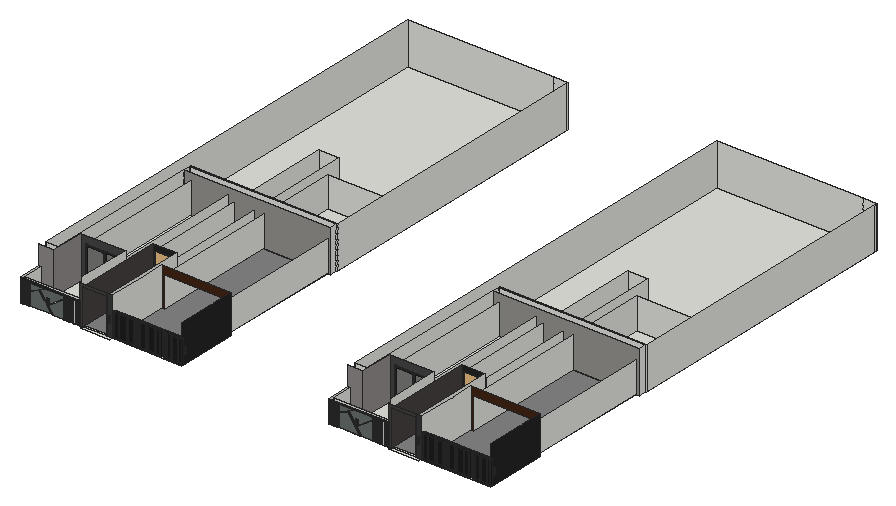
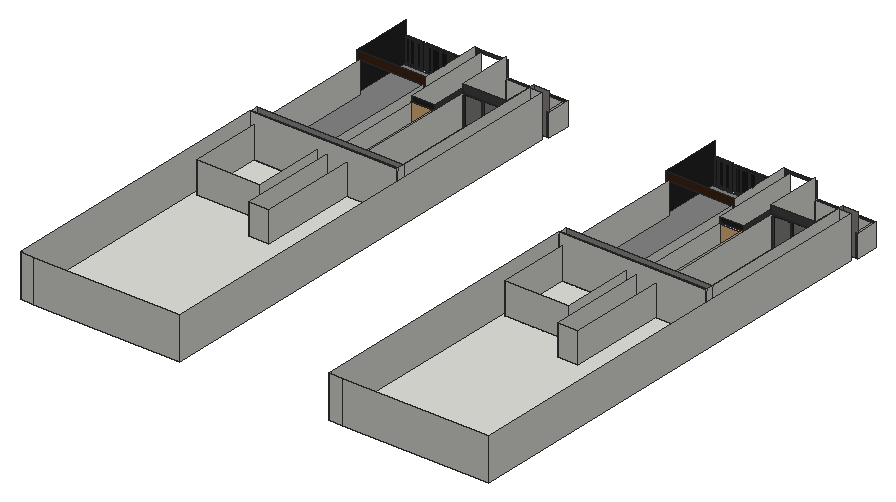
# SketchUp Ruby script. Lengths in inches.
U = 1.inch
M = Sketchup.active_model
def pt(a) = Geom::Point3d.new(a.map { |v| v * U })
def face(e, loops, mat)
  f = e.add_face(loops[0].map { |a| pt(a) })
  loops[1..].each { |l| e.add_face(l.map { |a| pt(a) }).erase! }
  f.material = f.back_material = mat if mat
  f
end
# faces: each face lists its corners as indices into pts; further lists are holes
def faces(e, pts, list, mat = nil) = list.each { |f| face(e, (f[0].is_a?(Array) ? f : [f]).map { |l| l.map { |i| pts[i] } }, mat) }
# xy, xz, yz: faces in a plane at the given z, y or x. An outline is a flat list of corners, or four numbers for a rectangle; further outlines are holes
def ring(l) = l.size == 4 ? [[l[0], l[1]], [l[2], l[1]], [l[2], l[3]], [l[0], l[3]]] : l.each_slice(2).to_a
def flat(e, list, mat, &to3) = list.each { |f| face(e, (f[0].is_a?(Array) ? f : [f]).map { |l| ring(l).map { |u, v| to3.(u, v) } }, mat) }
def xy(e, z, list, mat = nil) = flat(e, list, mat) { |x, y| [x, y, z] }
def xz(e, y, list, mat = nil) = flat(e, list, mat) { |x, z| [x, y, z] }
def yz(e, x, list, mat = nil) = flat(e, list, mat) { |y, z| [x, y, z] }
def lines(e, pts, list) = list.each { |a, b| e.add_line(pt(pts[a]), pt(pts[b])) }
# prism: a flat outline (further loops are holes) pulled along v
def prism(e, loops, v, mat = nil)
  f = face(e, loops, mat); d = Geom::Vector3d.new(v.map { |x| x * U })
  f.pushpull(f.normal.samedirection?(d) ? d.length : -d.length)
end
def box(e, o, s, mat = nil) = prism(e, [[o, [o[0] + s[0], o[1], o[2]], [o[0] + s[0], o[1] + s[1], o[2]], [o[0], o[1] + s[1], o[2]]]], [0, 0, s[2]], mat)
def at(x, y, z, deg = 0) = Geom::Transformation.translation(pt([x, y, z])) * Geom::Transformation.rotation(ORIGIN, Z_AXIS, deg.degrees)
def axes(o, x, y, z) = Geom::Transformation.new([*x, 0, *y, 0, *z, 0, *pt(o).to_a, 1])
def part(name) = M.definitions.add(name)
# library, detail: a bought-in or finely detailed component or shape, given as its bounding box
def library(name, o, s) = part(name).tap { |d| box(d.entities, o, s) }
def detail(e, o, s) = box(e.add_group.entities, o, s)
def put(e, d, t, mat = nil) = e.add_instance(d, t).tap { |i| i.material = mat if mat }
def group(e, t, mat = nil) = e.add_group.tap { |g| g.transformation = t; g.material = mat if mat }.entities
root = M.entities
M.materials.add("Glass_Tinted_Gray").color = [0, 0, 0]
M.materials["Glass_Tinted_Gray"].alpha = 0.125
M.materials.add("[0135_DarkGray]").color = [81, 81, 81]
M.materials.add("[Color M07]").color = [58, 58, 58]
M.materials.add("[Color M08]").color = [30, 30, 30]
M.materials.add("[Granite Dark Gray]").color = [38, 37, 37]
M.materials.add("[Granite Dark Gray]1").color = [69, 68, 68]
M.materials.add("[Granite Light Gray]").color = [149, 148, 144]
M.materials.add("[Granite Tile]1").color = [68, 65, 63]
M.materials.add("[Mirror 02]").color = [229, 229, 229]
M.materials.add("[Slate]").color = [102, 110, 108]
M.materials.add("[Stone Marble]").color = [143, 138, 136]
M.materials.add("[Terrazzo Light Blue]").color = [196, 214, 227]
M.materials.add("[Tile Grey]").color = [132, 132, 132]
M.materials.add("[Wood Veneer 01]").color = [66, 38, 20]
c1 = part("Group\#7")
xy(c1.entities,0,[[6,0,4.45,0.2,3,0.8,1.76,1.76,0.8,3,0.2,4.45,0,6,0.2,7.55,0.8,9,1.76,10.24,3,11.2,4.45,11.8,6,12,7.55,11.8,9,11.2,10.24,10.24,11.2,9,11.8,7.55,12,6,11.8,4.45,11.2,3,10.24,1.76,9,0.8,7.55,0.2]])
xy(c1.entities,37,[[6,0,7.55,0.2,9,0.8,10.24,1.76,11.2,3,11.8,4.45,12,6,11.8,7.55,11.2,9,10.24,10.24,9,11.2,7.55,11.8,6,12,4.45,11.8,3,11.2,1.76,10.24,0.8,9,0.2,7.55,0,6,0.2,4.45,0.8,3,1.76,1.76,3,0.8,4.45,0.2]],"[Granite Tile]1")
p = [[4.45,0.2,0],[6,0,0],[6,0,37],[4.45,0.2,37],[7.55,0.2,0],[7.55,0.2,37],
  [3,0.8,0],[3,0.8,37],[9,0.8,0],[9,0.8,37],[1.76,1.76,0],[1.76,1.76,37],
  [10.24,1.76,0],[10.24,1.76,37],[0.8,3,0],[0.8,3,37],[11.2,3,0],[11.2,3,37],
  [0.2,4.45,0],[0.2,4.45,37],[11.8,4.45,0],[11.8,4.45,37],[0,6,0],[0,6,37],
  [12,6,0],[12,6,37],[0.2,7.55,0],[0.2,7.55,37],[11.8,7.55,0],[11.8,7.55,37],
  [0.8,9,0],[0.8,9,37],[11.2,9,0],[11.2,9,37],[1.76,10.24,0],[1.76,10.24,37],
  [10.24,10.24,0],[10.24,10.24,37],[3,11.2,0],[3,11.2,37],[9,11.2,0],[9,11.2,37],
  [4.45,11.8,0],[4.45,11.8,37],[7.55,11.8,0],[7.55,11.8,37],[6,12,0],[6,12,37]]
faces(c1.entities,p,[[0,1,2,3],[1,4,5,2],[6,0,3,7],[4,8,9,5],[10,6,7,11],[8,12,13,9],[14,10,11,15],[12,16,17,13],
  [18,14,15,19],[16,20,21,17],[22,18,19,23],[20,24,25,21],[26,22,23,27],[24,28,29,25],[30,26,27,31],[28,32,33,29],
  [34,30,31,35],[32,36,37,33],[38,34,35,39],[36,40,41,37],[42,38,39,43],[40,44,45,41],[46,42,43,47],[44,46,47,45]],"[Granite Tile]1")
c2 = part("PENTEK_RP Fineline 50S_Sliding_DoorCase_E1")
box(c2.entities,[0,0,0],[1.51,3.66,99.27],"[0135_DarkGray]")
c3 = part("PENTEK_RP Fineline 50S_SlidingDooe_Case_E2")
box(c3.entities,[0,0,0],[96.25,3.66,1.51],"[0135_DarkGray]")
c4 = part("pentek_RP Fineline 50S_SlidingDoor_Case")
put(c4.entities,c2,at(97.76,0,0))
put(c4.entities,c3,at(1.51,0,0))
put(c4.entities,c2,at(0,0,0))
put(c4.entities,c3,at(1.51,0,97.76))
c5 = part("PENTEK_RP Fineline 50S_SlidingDoor_GlazingBead_2")
box(c5.entities,[0,0,0],[0.56,0.59,94.39],"[0135_DarkGray]")
c6 = part("PENTEK_RP Fineline 50S_SlidingDoor_Glass")
box(c6.entities,[0,0,0],[46.58,0.16,94.39],"Glass_Tinted_Gray")
c7 = part("PENTEK_RP Fineline 50S_SlidingDoor_GlazingBead")
box(c7.entities,[0,0,0],[45.47,0.59,0.56],"[0135_DarkGray]")
c8 = part("PENTEK_RP Fineline 50S_SlidingDoor_Leaf_E1")
xy(c8.entities,0,[[0,0,0.93,1.97],[0.93,1.57,1.49,1.97]],"[0135_DarkGray]")
xy(c8.entities,96.25,[[0,0,0.93,0,0.93,1.57,1.49,1.57,1.49,1.97,0,1.97]],"[0135_DarkGray]")
xz(c8.entities,0,[[0,0,0.93,96.25]],"[0135_DarkGray]")
xz(c8.entities,1.57,[[0.93,0,1.49,95.32],[0.93,95.32,1.49,96.25]],"[0135_DarkGray]")
xz(c8.entities,1.97,[[0,0,1.49,96.25]],"[0135_DarkGray]")
yz(c8.entities,0,[[0,0,1.97,96.25]],"[0135_DarkGray]")
yz(c8.entities,0.93,[[0,0,1.57,0.93],[0,0.93,1.57,95.32],[0,95.32,1.57,96.25]],"[0135_DarkGray]")
yz(c8.entities,1.49,[[1.57,0,1.97,95.32],[1.57,95.32,1.97,96.25]],"[0135_DarkGray]")
c9 = part("PENTEK_RP Fineline 50S_SlidingDoor_Leaf_E2")
xy(c9.entities,0,[[0,0,0,1.57,0.56,1.57,0.56,1.97,46.02,1.97,46.02,1.57,46.58,1.57,46.58,0]],"[0135_DarkGray]")
xy(c9.entities,0.93,[[0,0,46.58,1.57]],"[0135_DarkGray]")
xy(c9.entities,1.49,[[0.56,1.57,46.02,1.97]],"[0135_DarkGray]")
xz(c9.entities,0,[[0,0,46.58,0.93]],"[0135_DarkGray]")
xz(c9.entities,1.57,[[0,0,0.56,0.93],[46.02,0,46.58,0.93],[0.56,0.93,46.02,1.49]],"[0135_DarkGray]")
xz(c9.entities,1.97,[[0.56,0,46.02,1.49]],"[0135_DarkGray]")
yz(c9.entities,0,[[0,0,1.57,0.93]],"[0135_DarkGray]")
yz(c9.entities,0.56,[[1.57,0,1.97,0.93],[1.57,0.93,1.97,1.49]],"[0135_DarkGray]")
yz(c9.entities,46.02,[[1.57,0,1.97,0.93],[1.57,0.93,1.97,1.49]],"[0135_DarkGray]")
yz(c9.entities,46.58,[[0,0,1.57,0.93]],"[0135_DarkGray]")
c10 = part("PENTEK_RP Fineline S_SlidingDoor_Leaf1")
put(c10.entities,c5,at(0.93,0,0.93))
put(c10.entities,c5,at(46.96,0,0.93))
put(c10.entities,c6,at(1.49,1.42,0.93))
put(c10.entities,c7,at(1.49,0,0.93))
put(c10.entities,c6,at(1.49,0.59,0.93),"[Terrazzo Light Blue]")
put(c10.entities,c8,at(0,0,0))
put(c10.entities,c8,axes([48.44,0,0],[-1,0,0],[0,1,0],[0,0,1]))
put(c10.entities,c9,axes([0.93,0,96.25],[1,0,0],[0,1,0],[0,0,-1]))
put(c10.entities,c9,at(0.93,0,0))
put(c10.entities,c7,at(1.49,0,94.77))
c11 = part("PENTEK_RP Fineline 50S_SlidingDoor_Leaf2")
put(c11.entities,c6,at(1.49,1.42,0.93))
put(c11.entities,c7,at(1.49,0,94.77))
put(c11.entities,c5,at(46.96,0,0.93))
put(c11.entities,c6,at(1.49,0.59,0.93),"[Mirror 02]")
put(c11.entities,c5,at(0.93,0,0.93))
put(c11.entities,c8,at(0,0,0))
put(c11.entities,c8,axes([48.44,0,0],[-1,0,0],[0,1,0],[0,0,1]))
put(c11.entities,c7,at(1.49,0,0.93))
put(c11.entities,c9,axes([0.93,0,96.25],[1,0,0],[0,1,0],[0,0,-1]))
put(c11.entities,c9,at(0.93,0,0))
c12 = part("PENTEK - Slimmest Steel Sliding Door / Window\#1")
put(c12.entities,c4,at(0,-1.88,-0.09))
put(c12.entities,c10,at(1.51,-2.27,1.42))
put(c12.entities,c11,at(49.32,-0.3,1.42))
c13 = library("元件\#5",[-4.39,0,0],[5.37,35.83,90.55])
c14 = part("Group\#102")
g1 = group(c14.entities,at(0,0,0))
prism(g1,[[[0,3,72],[70.5,3,72],[70.5,3,0],[0,3,0]],[[67.5,3,3],[67.5,3,69],[3,3,69],[3,3,3]]],[0,-3,0])
c15 = part("Group\#135")
box(c15.entities,[0,0,0],[0.5,1,66])
c16 = part("Group\#148")
box(c16.entities,[0,-1,0],[5.5,1,66])
box(c16.entities,[50.84,-1,0],[13.66,1,66])
box(c16.entities,[28.06,-1,0],[22.28,1,66])
box(c16.entities,[24.66,-1,0],[2.9,1,66])
box(c16.entities,[6,-1,0],[18.16,1,66])
c17 = part("Component\#23")
g2 = group(c17.entities,at(70.5,0,0),"[Color M08]")
put(g2,c14,axes([70.5,0,0],[-1,0,0],[0,1,0],[0,0,1]))
g3 = group(g2,at(3,2,3))
g4 = group(g3,at(0,-1,0))
box(g4,[0,0,0],[5.5,1,66])
box(g4,[50.84,0,0],[13.66,1,66])
box(g4,[28.06,0,0],[22.28,1,66])
box(g4,[24.66,0,0],[2.9,1,66])
box(g4,[6,0,0],[18.16,1,66])
put(g3,c15,axes([50.34,0,0],[1,0,0],[0,-1,0],[0,0,1]))
put(g3,c15,axes([24.16,0,0],[1,0,0],[0,-1,0],[0,0,1]))
put(g3,c15,axes([27.56,0,0],[1,0,0],[0,-1,0],[0,0,1]))
put(g3,c15,axes([5.5,0,0],[1,0,0],[0,-1,0],[0,0,1]))
g5 = group(c17.entities,at(70.5,0,0),"[Color M08]")
put(g5,c14,at(-70.5,0,0))
g6 = group(g5,at(-3,2,3,-180))
put(g6,c16,at(0,1,0))
put(g6,c15,at(50.34,0,0))
put(g6,c15,at(24.16,0,0))
put(g6,c15,at(27.56,0,0))
put(g6,c15,at(5.5,0,0))
g7 = group(c17.entities,at(150,0,0),"[Color M08]")
put(g7,c14,axes([54,0,0],[-0.76596,0,0],[0,1,0],[0,0,1]))
g8 = group(g7,at(2.3,2,3))
put(g8,c16,axes([0,-1,0],[0.76596,0,0],[0,-1,0],[0,0,1]))
put(g8,c15,axes([38.55,0,0],[0.76596,0,0],[0,-1,0],[0,0,1]))
put(g8,c15,axes([18.5,0,0],[0.76596,0,0],[0,-1,0],[0,0,1]))
put(g8,c15,axes([21.11,0,0],[0.76596,0,0],[0,-1,0],[0,0,1]))
put(g8,c15,axes([4.22,0,0],[0.76596,0,0],[0,-1,0],[0,0,1]))
xy(root,8.5,[[395.95,2285.625,480.15,2294.125],[1274.7,2285.625,1358.9,2294.125],[218.97,2293.1875,222.53,2294.125],[223.78,2293.1875,227.34,2294.125],[228.6,2293.1875,232.16,2294.125],
  [233.41,2293.1875,236.97,2294.125],[238.22,2293.1875,241.78,2294.125],[243.03,2293.1875,246.59,2294.125],[343.47,2293.1875,347.43,2294.125],[348.47,2293.1875,352.43,2294.125],
  [353.47,2293.1875,357.43,2294.125],[358.47,2293.1875,362.43,2294.125],[363.47,2293.1875,367.43,2294.125],[368.47,2293.1875,372.43,2294.125],[378.2,2293.1875,381.86,2294.125],
  [385.66,2293.1875,388.78,2294.125],[1097.72,2293.1875,1101.28,2294.125],[1102.53,2293.1875,1106.09,2294.125],[1107.35,2293.1875,1110.91,2294.125],[1112.16,2293.1875,1115.72,2294.125],
  [1116.97,2293.1875,1120.53,2294.125],[1121.78,2293.1875,1125.34,2294.125],[1222.22,2293.1875,1226.18,2294.125],[1227.22,2293.1875,1231.18,2294.125],[1232.22,2293.1875,1236.18,2294.125],
  [1237.22,2293.1875,1241.18,2294.125],[1242.22,2293.1875,1246.18,2294.125],[1247.22,2293.1875,1251.18,2294.125],[1256.95,2293.1875,1260.61,2294.125],[1264.41,2293.1875,1267.53,2294.125],
  [218.97,2294.125,218.97,2358.81,225.79,2358.81,225.79,2300.94,388.78,2300.94,388.78,2294.125,310.12,2294.125,310.12,2297,306.57,2297,306.57,2294.125],[306.57,2294.125,310.12,2297],[395.95,2294.125,463.7,2300.94],[481.29,2294.125,678.9,2300.94],[1097.72,2294.125,1097.72,2358.81,1104.54,2358.81,1104.54,2300.94,1267.53,2300.94,1267.53,2294.125,1188.87,2294.125,1188.87,2297,1185.32,2297,1185.32,2294.125],
  [1185.32,2294.125,1188.87,2297],[1274.7,2294.125,1342.45,2300.94],[1360.04,2294.125,1557.65,2300.94],[225.79,2300.94,388.78,2300.94,388.78,2454.68,262.66,2454.68,262.66,2358.81,225.79,2358.81],[1104.54,2300.94,1267.53,2300.94,1267.53,2454.68,1141.41,2454.68,1141.41,2358.81,1104.54,2358.81],
  [225.79,2374.65,261.53,2374.65,261.53,2846.52,402.97,2846.52,402.97,3124.06,460.85,3124.06,460.85,2846.52,488.9,2846.52,488.9,3049.31,669.8,3049.31,669.8,2846.52,678.9,2846.52,678.9,3664.43,225.79,3664.43],[1104.54,2374.65,1140.28,2374.65,1140.28,2846.52,1281.72,2846.52,1281.72,3124.06,1339.6,3124.06,1339.6,2846.52,1367.65,2846.52,1367.65,3049.31,1548.55,3049.31,1548.55,2846.52,1557.65,2846.52,1557.65,3664.43,1104.54,3664.43],[261.53,2822.08,402.97,2841.77],[402.97,2822.08,460.85,2841.77],[460.85,2822.08,488.9,2841.77],
  [488.9,2822.08,669.8,2841.77],[669.8,2822.08,678.9,2841.77],[1140.28,2822.08,1281.72,2841.77],[1281.72,2822.08,1339.6,2841.77],[1339.6,2822.08,1367.65,2841.77],
  [1367.65,2822.08,1548.55,2841.77],[1548.55,2822.08,1557.65,2841.77],[261.53,2841.77,402.97,2846.52],[402.97,2841.77,460.85,2846.52],[460.85,2841.77,488.9,2846.52],
  [488.9,2841.77,669.8,2846.52],[669.8,2841.77,678.9,2846.52],[1140.28,2841.77,1281.72,2846.52],[1281.72,2841.77,1339.6,2846.52],[1339.6,2841.77,1367.65,2846.52],
  [1367.65,2841.77,1548.55,2846.52],[1548.55,2841.77,1557.65,2846.52],[402.97,2846.52,460.85,3124.06],[488.9,2846.52,669.8,3049.31],[1281.72,2846.52,1339.6,3124.06],
  [1367.65,2846.52,1548.55,3049.31]])
xy(root,8.5,[[395.95,2300.94,463.7,2300.94,463.7,2542.24,460.85,2542.24,460.85,2822.08,402.97,2822.08,402.97,2542.24,395.95,2542.24],[481.29,2300.94,678.9,2300.94,678.9,2468.68,669.8,2468.68,669.8,2822.08,488.9,2822.08,488.9,2468.68,481.29,2468.68],[1274.7,2300.94,1342.45,2300.94,1342.45,2542.24,1339.6,2542.24,1339.6,2822.08,1281.72,2822.08,1281.72,2542.24,1274.7,2542.24],[1360.04,2300.94,1557.65,2300.94,1557.65,2468.68,1548.55,2468.68,1548.55,2822.08,1367.65,2822.08,1367.65,2468.68,1360.04,2468.68]],"[Tile Grey]")
xy(root,20.01,[[279.88,2454.68,385.01,2841.77],[1158.63,2454.68,1263.76,2841.77]])
xy(root,68.78,[[222.53,2293.1875,223.78,2294.125],[227.34,2293.1875,228.6,2294.125],[232.16,2293.1875,233.41,2294.125],[236.97,2293.1875,238.22,2294.125],[241.78,2293.1875,243.03,2294.125],
  [246.59,2293.1875,246.59,2294.125,290.35,2294.125,290.35,2297,293.48,2297,293.48,2294.125,343.47,2294.125,343.47,2293.1875],[347.43,2293.1875,348.47,2294.125],[352.43,2293.1875,353.47,2294.125],[357.43,2293.1875,358.47,2294.125],[362.43,2293.1875,363.47,2294.125],
  [367.43,2293.1875,368.47,2294.125],[372.43,2293.1875,378.2,2294.125],[381.86,2293.1875,385.66,2294.125],[1101.28,2293.1875,1102.53,2294.125],[1106.09,2293.1875,1107.35,2294.125],
  [1110.91,2293.1875,1112.16,2294.125],[1115.72,2293.1875,1116.97,2294.125],[1120.53,2293.1875,1121.78,2294.125],[1125.34,2293.1875,1125.34,2294.125,1169.1,2294.125,1169.1,2297,1172.23,2297,1172.23,2294.125,1222.22,2294.125,1222.22,2293.1875],[1226.18,2293.1875,1227.22,2294.125],
  [1231.18,2293.1875,1232.22,2294.125],[1236.18,2293.1875,1237.22,2294.125],[1241.18,2293.1875,1242.22,2294.125],[1246.18,2293.1875,1247.22,2294.125],[1251.18,2293.1875,1256.95,2294.125],
  [1260.61,2293.1875,1264.41,2294.125]])
xz(root,2293.1875,[[218.97,8.5,222.53,68.78],[223.78,8.5,227.34,68.78],[228.6,8.5,232.16,68.78],[233.41,8.5,236.97,68.78],[238.22,8.5,241.78,68.78],
  [243.03,8.5,246.59,68.78],[343.47,8.5,347.43,68.78],[348.47,8.5,352.43,68.78],[353.47,8.5,357.43,68.78],[358.47,8.5,362.43,68.78],
  [363.47,8.5,367.43,68.78],[385.66,8.5,388.78,68.78],[1097.72,8.5,1101.28,68.78],[1102.53,8.5,1106.09,68.78],[1107.35,8.5,1110.91,68.78],
  [1112.16,8.5,1115.72,68.78],[1116.97,8.5,1120.53,68.78],[1121.78,8.5,1125.34,68.78],[1222.22,8.5,1226.18,68.78],[1227.22,8.5,1231.18,68.78],
  [1232.22,8.5,1236.18,68.78],[1237.22,8.5,1241.18,68.78],[1242.22,8.5,1246.18,68.78],[1264.41,8.5,1267.53,68.78],[218.97,68.78,388.78,72.4375],
  [1097.72,68.78,1267.53,72.4375]],"[Color M08]")
xz(root,2293.1875,[[368.47,8.5,372.43,68.78],[378.2,8.5,381.86,68.78],[1247.22,8.5,1251.18,68.78],[1256.95,8.5,1260.61,68.78]],"[Slate]")
xz(root,2294.125,[[222.53,8.5,223.78,68.78],[227.34,8.5,228.6,68.78],[232.16,8.5,233.41,68.78],[236.97,8.5,238.22,68.78],[241.78,8.5,243.03,68.78],
  [347.43,8.5,348.47,68.78],[352.43,8.5,353.47,68.78],[357.43,8.5,358.47,68.78],[362.43,8.5,363.47,68.78],[367.43,8.5,368.47,68.78],
  [1101.28,8.5,1102.53,68.78],[1106.09,8.5,1107.35,68.78],[1110.91,8.5,1112.16,68.78],[1115.72,8.5,1116.97,68.78],[1120.53,8.5,1121.78,68.78],
  [1226.18,8.5,1227.22,68.78],[1231.18,8.5,1232.22,68.78],[1236.18,8.5,1237.22,68.78],[1241.18,8.5,1242.22,68.78],[1246.18,8.5,1247.22,68.78]])
xz(root,2294.125,[[463.7,8.5,481.29,118.38],[1342.45,8.5,1360.04,118.38]],"[Color M07]")
xz(root,2294.125,[[372.43,8.5,378.2,68.78],[381.86,8.5,385.66,68.78],[1251.18,8.5,1256.95,68.78],[1260.61,8.5,1264.41,68.78]],"[Color M08]")
xz(root,2294.125,[[388.78,8.5,395.95,8.5,395.95,110.32,463.7,110.32,463.7,118.38,388.78,118.38],[1267.53,8.5,1274.7,8.5,1274.7,110.32,1342.45,110.32,1342.45,118.38,1267.53,118.38]],"[Granite Tile]1")
xz(root,2294.125,[[246.59,8.5,306.57,8.5,271.87,57.375,246.59,44.04],[310.12,8.5,343.47,8.5,343.47,58.8,297.81,25.91],[1125.34,8.5,1185.32,8.5,1150.62,57.375,1125.34,44.04],[1188.87,8.5,1222.22,8.5,1222.22,58.8,1176.56,25.91],[295.39,29.34,343.47,62.06,343.47,68.78,293.48,68.78,274.57,58.8],
  [1174.14,29.34,1222.22,62.06,1222.22,68.78,1172.23,68.78,1153.32,58.8],[246.59,46.32,290.35,68.78,246.59,68.78],[1125.34,46.32,1169.1,68.78,1125.34,68.78]],"[Slate]")
xz(root,2297,[[306.57,8.5,310.12,8.5,297.81,25.91,295.39,29.34,274.57,58.8,271.87,57.375],[1185.32,8.5,1188.87,8.5,1176.56,25.91,1174.14,29.34,1153.32,58.8,1150.62,57.375],[297.81,25.91,343.47,58.8,343.47,62.06,295.39,29.34],[1176.56,25.91,1222.22,58.8,1222.22,62.06,1174.14,29.34],[246.59,44.04,271.87,57.375,274.57,58.8,293.48,68.78,290.35,68.78,246.59,46.32],
  [1125.34,44.04,1150.62,57.375,1153.32,58.8,1172.23,68.78,1169.1,68.78,1125.34,46.32]])
xz(root,2300.94,[[225.79,8.5,388.78,72.4375],[1104.54,8.5,1267.53,72.4375]])
xz(root,2358.81,[[218.97,8.5,225.79,72.4375],[1097.72,8.5,1104.54,72.4375]])
xz(root,2358.81,[[225.79,8.5,262.66,8.5,262.66,128.5,218.97,128.5,218.97,72.4375,225.79,72.4375],[1104.54,8.5,1141.41,8.5,1141.41,128.5,1097.72,128.5,1097.72,72.4375,1104.54,72.4375]],"[Stone Marble]")
xz(root,2374.65,[[225.79,8.5,261.53,128.5],[1104.54,8.5,1140.28,128.5]])
xz(root,2454.68,[[[262.66,8.5,388.78,128.5],[279.88,20.01,385.01,107.07]],[[1141.41,8.5,1267.53,128.5],[1158.63,20.01,1263.76,107.07]]],"[Granite Dark Gray]1")
xz(root,2468.68,[[481.29,8.5,488.9,8.5,488.9,96.29,669.8,96.29,669.8,8.5,678.9,8.5,678.9,118.38,481.29,118.38],[1360.04,8.5,1367.65,8.5,1367.65,96.29,1548.55,96.29,1548.55,8.5,1557.65,8.5,1557.65,118.38,1360.04,118.38]],"[Wood Veneer 01]")
xz(root,2542.24,[[395.95,8.5,402.97,8.5,402.97,96.1875,460.85,96.1875,460.85,8.5,463.7,8.5,463.7,110.32,395.95,110.32],[1274.7,8.5,1281.72,8.5,1281.72,96.1875,1339.6,96.1875,1339.6,8.5,1342.45,8.5,1342.45,110.32,1274.7,110.32]],"[Granite Dark Gray]")
xz(root,2822.08,[[261.53,8.5,678.9,128.5],[1140.28,8.5,1557.65,128.5]],"[Granite Light Gray]")
xz(root,2841.77,[[[261.53,8.5,678.9,128.5],[279.88,20.01,385.01,107.07]],[[1140.28,8.5,1557.65,128.5],[1158.63,20.01,1263.76,107.07]]])
xz(root,2846.52,[[261.53,8.5,678.9,128.5],[1140.28,8.5,1557.65,128.5]])
xz(root,3049.31,[[488.9,8.5,669.8,96.29],[1367.65,8.5,1548.55,96.29]])
xz(root,3124.06,[[402.97,8.5,460.85,96.1875],[1281.72,8.5,1339.6,96.1875]])
xz(root,3664.43,[[225.79,8.5,640.4,128.5],[640.4,8.5,678.9,128.5],[1104.54,8.5,1519.15,128.5],[1519.15,8.5,1557.65,128.5]])
yz(root,218.97,[[2293.1875,8.5,2358.81,72.4375]])
yz(root,222.53,[[2293.1875,8.5,2294.125,68.78]])
yz(root,223.78,[[2293.1875,8.5,2294.125,68.78]])
yz(root,225.79,[[2300.94,8.5,2358.81,72.4375],[2374.65,8.5,3664.43,128.5]])
yz(root,227.34,[[2293.1875,8.5,2294.125,68.78]])
yz(root,228.6,[[2293.1875,8.5,2294.125,68.78]])
yz(root,232.16,[[2293.1875,8.5,2294.125,68.78]])
yz(root,233.41,[[2293.1875,8.5,2294.125,68.78]])
yz(root,236.97,[[2293.1875,8.5,2294.125,68.78]])
yz(root,238.22,[[2293.1875,8.5,2294.125,68.78]])
yz(root,241.78,[[2293.1875,8.5,2294.125,68.78]])
yz(root,243.03,[[2293.1875,8.5,2294.125,68.78]])
yz(root,246.59,[[2293.1875,8.5,2294.125,8.5,2294.125,44.04,2297,44.04,2297,46.32,2294.125,46.32,2294.125,68.78,2293.1875,68.78]])
yz(root,261.53,[[2374.65,8.5,2822.08,128.5],[2822.08,8.5,2841.77,128.5],[2841.77,8.5,2846.52,128.5]])
yz(root,262.66,[[2358.81,8.5,2454.68,128.5]],"[Stone Marble]")
yz(root,279.88,[[2454.68,20.01,2841.77,107.07]])
yz(root,343.47,[[2293.1875,8.5,2293.1875,68.78,2294.125,68.78,2294.125,62.06,2297,62.06,2297,58.8,2294.125,58.8,2294.125,8.5]])
yz(root,347.43,[[2293.1875,8.5,2294.125,68.78]])
yz(root,348.47,[[2293.1875,8.5,2294.125,68.78]])
yz(root,352.43,[[2293.1875,8.5,2294.125,68.78]])
yz(root,353.47,[[2293.1875,8.5,2294.125,68.78]])
yz(root,357.43,[[2293.1875,8.5,2294.125,68.78]])
yz(root,358.47,[[2293.1875,8.5,2294.125,68.78]])
yz(root,362.43,[[2293.1875,8.5,2294.125,68.78]])
yz(root,363.47,[[2293.1875,8.5,2294.125,68.78]])
yz(root,367.43,[[2293.1875,8.5,2294.125,68.78]])
yz(root,368.47,[[2293.1875,8.5,2294.125,68.78]])
yz(root,372.43,[[2293.1875,8.5,2294.125,68.78]])
yz(root,378.2,[[2293.1875,8.5,2294.125,68.78]])
yz(root,381.86,[[2293.1875,8.5,2294.125,68.78]])
yz(root,385.01,[[2454.68,20.01,2841.77,107.07]])
yz(root,385.66,[[2293.1875,8.5,2294.125,68.78]])
yz(root,388.78,[[2293.1875,8.5,2294.125,68.78],[2294.125,8.5,2300.94,72.4375],[2300.94,8.5,2454.68,128.5],[2293.1875,68.78,2294.125,72.4375]])
yz(root,395.95,[[2294.125,8.5,2542.24,110.32]],"[Granite Tile]1")
yz(root,402.97,[[2542.24,8.5,3124.06,96.1875]])
yz(root,460.85,[[2542.24,8.5,3124.06,96.1875]])
yz(root,463.7,[[2294.125,8.5,2542.24,110.32]])
yz(root,481.29,[[2294.125,8.5,2468.68,8.5,2468.68,118.38,2407.27,118.38,2407.27,116.94,2396.68,116.94,2396.68,118.38,2294.125,118.38]])
yz(root,488.9,[[2468.68,8.5,3049.31,96.29]])
yz(root,669.8,[[2468.68,8.5,3049.31,96.29]])
yz(root,678.9,[[2822.08,8.5,2841.77,128.5],[2841.77,8.5,2846.52,128.5],[2846.52,8.5,3658.44,128.5],[3658.44,8.5,3664.43,128.5]])
yz(root,678.9,[[2294.125,8.5,2294.125,118.38,2396.68,118.38,2396.68,116.94,2407.27,116.94,2407.27,118.38,2468.68,118.38,2468.68,8.5]],"[Granite Dark Gray]")
yz(root,1097.72,[[2293.1875,8.5,2358.81,72.4375]])
yz(root,1101.28,[[2293.1875,8.5,2294.125,68.78]])
yz(root,1102.53,[[2293.1875,8.5,2294.125,68.78]])
yz(root,1104.54,[[2300.94,8.5,2358.81,72.4375],[2374.65,8.5,3664.43,128.5]])
yz(root,1106.09,[[2293.1875,8.5,2294.125,68.78]])
yz(root,1107.35,[[2293.1875,8.5,2294.125,68.78]])
yz(root,1110.91,[[2293.1875,8.5,2294.125,68.78]])
yz(root,1112.16,[[2293.1875,8.5,2294.125,68.78]])
yz(root,1115.72,[[2293.1875,8.5,2294.125,68.78]])
yz(root,1116.97,[[2293.1875,8.5,2294.125,68.78]])
yz(root,1120.53,[[2293.1875,8.5,2294.125,68.78]])
yz(root,1121.78,[[2293.1875,8.5,2294.125,68.78]])
yz(root,1125.34,[[2293.1875,8.5,2294.125,8.5,2294.125,44.04,2297,44.04,2297,46.32,2294.125,46.32,2294.125,68.78,2293.1875,68.78]])
yz(root,1140.28,[[2374.65,8.5,2822.08,128.5],[2822.08,8.5,2841.77,128.5],[2841.77,8.5,2846.52,128.5]])
yz(root,1141.41,[[2358.81,8.5,2454.68,128.5]],"[Stone Marble]")
yz(root,1158.63,[[2454.68,20.01,2841.77,107.07]])
yz(root,1222.22,[[2293.1875,8.5,2293.1875,68.78,2294.125,68.78,2294.125,62.06,2297,62.06,2297,58.8,2294.125,58.8,2294.125,8.5]])
yz(root,1226.18,[[2293.1875,8.5,2294.125,68.78]])
yz(root,1227.22,[[2293.1875,8.5,2294.125,68.78]])
yz(root,1231.18,[[2293.1875,8.5,2294.125,68.78]])
yz(root,1232.22,[[2293.1875,8.5,2294.125,68.78]])
yz(root,1236.18,[[2293.1875,8.5,2294.125,68.78]])
yz(root,1237.22,[[2293.1875,8.5,2294.125,68.78]])
yz(root,1241.18,[[2293.1875,8.5,2294.125,68.78]])
yz(root,1242.22,[[2293.1875,8.5,2294.125,68.78]])
yz(root,1246.18,[[2293.1875,8.5,2294.125,68.78]])
yz(root,1247.22,[[2293.1875,8.5,2294.125,68.78]])
yz(root,1251.18,[[2293.1875,8.5,2294.125,68.78]])
yz(root,1256.95,[[2293.1875,8.5,2294.125,68.78]])
yz(root,1260.61,[[2293.1875,8.5,2294.125,68.78]])
yz(root,1263.76,[[2454.68,20.01,2841.77,107.07]])
yz(root,1264.41,[[2293.1875,8.5,2294.125,68.78]])
yz(root,1267.53,[[2293.1875,8.5,2294.125,68.78],[2294.125,8.5,2300.94,72.4375],[2300.94,8.5,2454.68,128.5],[2293.1875,68.78,2294.125,72.4375]])
yz(root,1274.7,[[2294.125,8.5,2542.24,110.32]],"[Granite Tile]1")
yz(root,1281.72,[[2542.24,8.5,3124.06,96.1875]])
yz(root,1339.6,[[2542.24,8.5,3124.06,96.1875]])
yz(root,1342.45,[[2294.125,8.5,2542.24,110.32]])
yz(root,1360.04,[[2294.125,8.5,2468.68,8.5,2468.68,118.38,2407.27,118.38,2407.27,116.94,2396.68,116.94,2396.68,118.38,2294.125,118.38]])
yz(root,1367.65,[[2468.68,8.5,3049.31,96.29]])
yz(root,1548.55,[[2468.68,8.5,3049.31,96.29]])
yz(root,1557.65,[[2822.08,8.5,2841.77,128.5],[2841.77,8.5,2846.52,128.5],[2846.52,8.5,3658.44,128.5],[3658.44,8.5,3664.43,128.5]])
yz(root,1557.65,[[2294.125,8.5,2294.125,118.38,2396.68,118.38,2396.68,116.94,2407.27,116.94,2407.27,118.38,2468.68,118.38,2468.68,8.5]],"[Granite Dark Gray]")
p = [[271.87,2294.125,57.375],[306.57,2294.125,8.5],[306.57,2297,8.5],[271.87,2297,57.375],[310.12,2294.125,8.5],[297.81,2294.125,25.91],
  [297.81,2297,25.91],[310.12,2297,8.5],[1150.62,2294.125,57.375],[1185.32,2294.125,8.5],[1185.32,2297,8.5],[1150.62,2297,57.375],
  [1188.87,2294.125,8.5],[1176.56,2294.125,25.91],[1176.56,2297,25.91],[1188.87,2297,8.5],[343.47,2294.125,58.8],[343.47,2297,58.8],
  [1222.22,2294.125,58.8],[1222.22,2297,58.8],[295.39,2294.125,29.34],[274.57,2294.125,58.8],[274.57,2297,58.8],[295.39,2297,29.34],
  [343.47,2294.125,62.06],[343.47,2297,62.06],[1174.14,2294.125,29.34],[1153.32,2294.125,58.8],[1153.32,2297,58.8],[1174.14,2297,29.34],
  [1222.22,2294.125,62.06],[1222.22,2297,62.06],[246.59,2294.125,44.04],[246.59,2297,44.04],[1125.34,2294.125,44.04],[1125.34,2297,44.04],
  [290.35,2294.125,68.78],[246.59,2294.125,46.32],[246.59,2297,46.32],[290.35,2297,68.78],[1169.1,2294.125,68.78],[1125.34,2294.125,46.32],
  [1125.34,2297,46.32],[1169.1,2297,68.78],[293.48,2294.125,68.78],[293.48,2297,68.78],[1172.23,2294.125,68.78],[1172.23,2297,68.78]]
faces(root,p,[[0,1,2,3],[4,5,6,7],[8,9,10,11],[12,13,14,15],[5,16,17,6],[13,18,19,14],[20,21,22,23],[24,20,23,25],
  [26,27,28,29],[30,26,29,31],[32,0,3,33],[34,8,11,35],[36,37,38,39],[40,41,42,43],[21,44,45,22],[27,46,47,28]])
put(root,c1,axes([294.35,2291.96,29.51],[0.42,0,0],[0,0.42,0],[0,0,0.42]))
put(root,c12,axes([276.88,2454.68,20],[1.08916,0,0],[0,1,0],[0,0,0.87793]))
put(root,c13,axes([402.97,2542.62,8.5],[0,-1,0],[1.61541,0,0],[0,0,0.96838]))
put(root,c1,axes([469.78,2289.08,47.16],[0.42,0,0],[0,0.42,0],[0,0,0.42]))
put(root,c17,axes([481.29,2294.125,8.5],[0.9687,0,0],[0,1,0],[0,0,1]))
put(root,c1,axes([685.86,2289.09,44.5],[0.42,0,0],[0,0.42,0],[0,0,0.42]))
put(root,c1,axes([1173.1,2291.96,29.51],[0.42,0,0],[0,0.42,0],[0,0,0.42]))
put(root,c12,axes([1155.63,2454.68,20],[1.08916,0,0],[0,1,0],[0,0,0.87793]))
put(root,c13,axes([1281.72,2542.62,8.5],[0,-1,0],[1.61541,0,0],[0,0,0.96838]))
put(root,c1,axes([1348.53,2289.08,47.16],[0.42,0,0],[0,0.42,0],[0,0,0.42]))
put(root,c17,axes([1360.04,2294.125,8.5],[0.9687,0,0],[0,1,0],[0,0,1]))
put(root,c1,axes([1564.61,2289.09,44.5],[0.42,0,0],[0,0.42,0],[0,0,0.42]))
